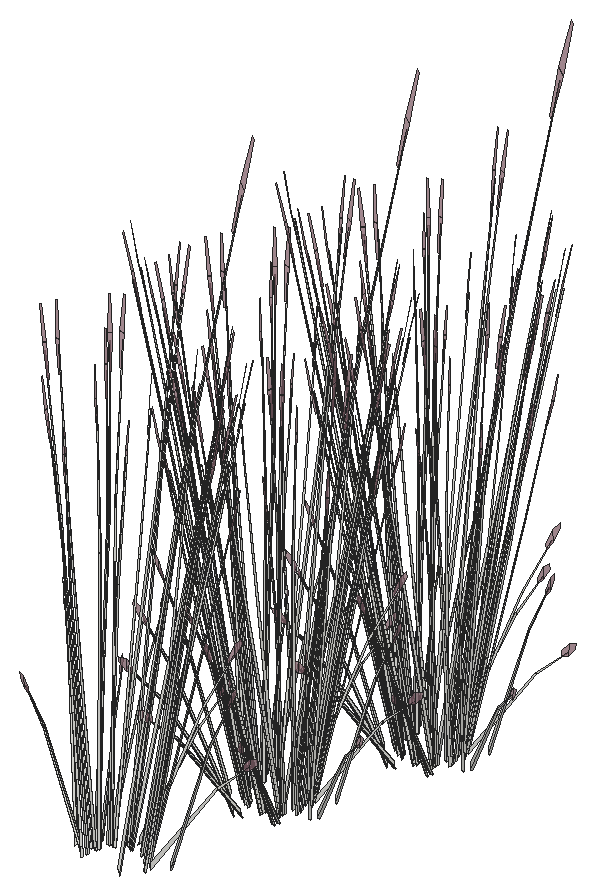
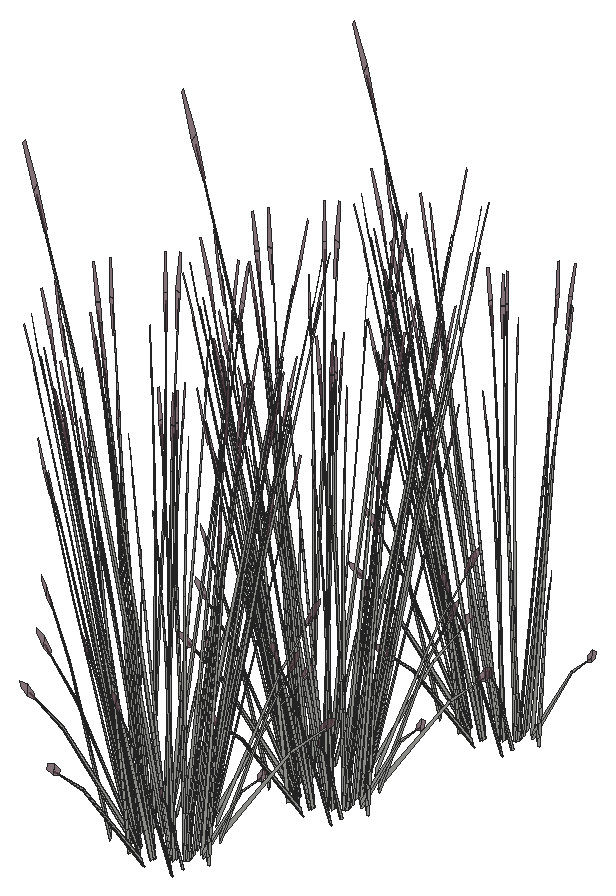
# SketchUp Ruby script. Lengths in inches.
U = 1.inch
M = Sketchup.active_model
def pt(a) = Geom::Point3d.new(a.map { |v| v * U })
def face(e, loops, mat)
  f = e.add_face(loops[0].map { |a| pt(a) })
  loops[1..].each { |l| e.add_face(l.map { |a| pt(a) }).erase! }
  f.material = f.back_material = mat if mat
  f
end
# faces: each face lists its corners as indices into pts; further lists are holes
def faces(e, pts, list, mat = nil) = list.each { |f| face(e, (f[0].is_a?(Array) ? f : [f]).map { |l| l.map { |i| pts[i] } }, mat) }
# xy, xz, yz: faces in a plane at the given z, y or x. An outline is a flat list of corners, or four numbers for a rectangle; further outlines are holes
def ring(l) = l.size == 4 ? [[l[0], l[1]], [l[2], l[1]], [l[2], l[3]], [l[0], l[3]]] : l.each_slice(2).to_a
def flat(e, list, mat, &to3) = list.each { |f| face(e, (f[0].is_a?(Array) ? f : [f]).map { |l| ring(l).map { |u, v| to3.(u, v) } }, mat) }
def xy(e, z, list, mat = nil) = flat(e, list, mat) { |x, y| [x, y, z] }
def xz(e, y, list, mat = nil) = flat(e, list, mat) { |x, z| [x, y, z] }
def yz(e, x, list, mat = nil) = flat(e, list, mat) { |y, z| [x, y, z] }
def lines(e, pts, list) = list.each { |a, b| e.add_line(pt(pts[a]), pt(pts[b])) }
# prism: a flat outline (further loops are holes) pulled along v
def prism(e, loops, v, mat = nil)
  f = face(e, loops, mat); d = Geom::Vector3d.new(v.map { |x| x * U })
  f.pushpull(f.normal.samedirection?(d) ? d.length : -d.length)
end
def box(e, o, s, mat = nil) = prism(e, [[o, [o[0] + s[0], o[1], o[2]], [o[0] + s[0], o[1] + s[1], o[2]], [o[0], o[1] + s[1], o[2]]]], [0, 0, s[2]], mat)
def at(x, y, z, deg = 0) = Geom::Transformation.translation(pt([x, y, z])) * Geom::Transformation.rotation(ORIGIN, Z_AXIS, deg.degrees)
def axes(o, x, y, z) = Geom::Transformation.new([*x, 0, *y, 0, *z, 0, *pt(o).to_a, 1])
def part(name) = M.definitions.add(name)
# library, detail: a bought-in or finely detailed component or shape, given as its bounding box
def library(name, o, s) = part(name).tap { |d| box(d.entities, o, s) }
def detail(e, o, s) = box(e.add_group.entities, o, s)
def put(e, d, t, mat = nil) = e.add_instance(d, t).tap { |i| i.material = mat if mat }
def group(e, t, mat = nil) = e.add_group.tap { |g| g.transformation = t; g.material = mat if mat }.entities
root = M.entities
M.materials.add("LightPink_Translucent").color = [144, 107, 117]
M.materials["LightPink_Translucent"].alpha = 0.75
c1 = part("blade")
p = [[2.15,0.21,22],[0,0.17,0],[0.09,0.45,0],[2.18,0.31,22],[2.29,0.31,22],[0.38,0.45,0],
  [2.48,0.24,33],[2.49,0.24,33],[2.48,0.22,33]]
faces(c1.entities,p,[[0,1,2,3],[4,5,2,3],[6,3,4,7],[8,0,3,6]])
c2 = part("seeds")
p = [[0.3,-0.1,1.38],[-0.01,-0.03,1.59],[-0.01,-0.03,0.03],[0.14,-0.07,-0.07],[0.29,-0.03,3],[0.15,0.01,3.11]]
faces(c2.entities,p,[[0,1,2,3],[1,0,4,5]],"LightPink_Translucent")
c3 = part("blade with seeds")
put(c3.entities,c1,at(0,0,0))
put(c3.entities,c2,axes([2.4,0.25,30.99],[1.5799,-0.05474,1.17369],[-0.12525,1.92788,0.29478],[-0.07173,-0.02425,1.56792]))
put(root,c3,axes([315.38,325.84,526.73],[-0.14195,0.49104,0.48003],[-0.46669,-0.16791,0.3958],[0.18353,-0.02951,0.9933]))
put(root,c3,axes([311.01,325.04,527.05],[0.41757,0.15024,0.35414],[-0.12179,0.4383,-0.4572],[-0.16812,0.04019,0.87481]))
put(root,c3,axes([316.22,327.43,526.71],[-0.04543,-0.04715,1.77383],[0.09938,-0.50538,-0.16761],[0.17896,-0.03229,0.31391]))
put(root,c3,axes([310.3,325.375,526.72],[-0.08205,0.06992,1.74944],[0.00698,0.51086,-0.27667],[-0.18807,0.06644,0.14031]))
put(root,c3,axes([310.83,324.89,527.03],[0.25281,0.48765,-0.1216],[-0.44869,0.23964,-0.67495],[-0.18908,0.06434,1.02557]))
put(root,c3,axes([314.64,326.99,527.03],[0.0269,-0.54769,-0.1216],[0.50939,0.01497,-0.67495],[0.19618,0.03804,1.02557]))
put(root,c3,axes([314.57,326.78,527.05],[-0.28589,-0.33718,0.35414],[0.32644,-0.31919,-0.4572],[0.16586,0.04856,0.87481]))
put(root,c3,axes([315.09,326.66,526.72],[0.10779,-0.00911,1.74944],[0.29564,-0.41839,-0.27667],[0.19172,0.05523,0.14031]))
put(root,c3,axes([310.78,326.25,526.73],[-0.12461,-0.49565,0.48003],[0.48882,-0.08602,0.3958],[-0.14406,0.11657,0.9933]))
put(root,c3,axes([310.68,326.16,526.73],[-0.34493,-0.22649,0.0643],[0.20082,-0.32253,0.50621],[-0.11059,0.10427,0.77189]))
put(root,c3,axes([311.08,326.09,527.05],[0.43736,-0.07697,0.35414],[0.11549,0.43998,-0.4572],[-0.12533,0.11818,0.87481]))
put(root,c3,axes([309.39,325.89,526.71],[0.06412,0.01444,1.77383],[0.19837,0.47583,-0.16761],[-0.13126,0.12489,0.31391]))
put(root,c3,axes([314.82,327.08,526.73],[-0.0253,0.40952,0.0643],[-0.38204,-0.01123,0.50621],[0.14634,0.04285,0.77189]))
put(root,c3,axes([314.86,326.95,526.73],[-0.37048,0.35486,0.48003],[-0.31952,-0.37685,0.3958],[0.17382,0.06546,0.9933]))
put(root,c3,axes([310.08,327.34,527.65],[0.44338,0.14375,-0.06488],[-0.13639,0.44245,-0.29416],[-0.07252,0.06718,0.97024]))
put(root,c3,axes([313.68,327.36,527.05],[-0.0776,-0.43378,0.35414],[0.44361,-0.11454,-0.4572],[0.11915,0.12431,0.87481]))
put(root,c3,axes([313.98,324.87,526.47],[-0.43417,-0.27982,1.38283],[0.45844,-0.43566,0.59665],[0.14008,0.26255,1.33663]))
put(root,c3,axes([310.85,326.05,527.03],[0.46478,0.29695,-0.1216],[-0.26776,0.43004,-0.67495],[-0.13131,0.14949,1.02557]))
put(root,c3,axes([313.64,327.59,527.03],[0.2994,-0.46097,-0.1216],[0.43359,0.26557,-0.67495],[0.15072,0.13024,1.02557]))
put(root,c3,axes([311.67,326.96,527.05],[0.33997,-0.28354,0.35414],[0.32182,0.32376,-0.4572],[-0.04897,0.1645,0.87481]))
put(root,c3,axes([313.25,327.97,526.71],[0.00149,-0.0652,1.77383],[0.43058,-0.28766,-0.16761],[0.14956,0.10267,0.31391]))
put(root,c3,axes([311.36,327.22,526.73],[-0.4129,-0.02509,0.0643],[0.01132,-0.37891,0.50621],[-0.04321,0.14514,0.77189]))
put(root,c3,axes([311.49,327.26,526.73],[-0.35779,-0.36745,0.48003],[0.37996,-0.3169,0.3958],[-0.066,0.17239,0.9933]))
put(root,c3,axes([312.62,327.43,527.05],[0.15148,-0.41415,0.35414],[0.44193,0.12079,-0.4572],[0.04052,0.16674,0.87481]))
put(root,c3,axes([313.75,327.75,526.73],[-0.22836,0.34211,0.0643],[-0.3252,-0.19918,0.50621],[0.10513,0.10968,0.77189]))
put(root,c3,axes([313.22,328.91,527.65],[0.34721,-0.30895,-0.06488],[0.31814,0.33837,-0.29416],[0.0224,0.09588,0.97024]))
put(root,c3,axes([313.85,327.66,526.73],[-0.49974,0.12359,0.48003],[-0.08673,-0.48481,0.3958],[0.11753,0.14288,0.9933]))
put(root,c3,axes([312.48,327.81,526.73],[-0.37023,0.18303,0.0643],[-0.18122,-0.33376,0.50621],[0.03575,0.14712,0.77189]))
put(root,c3,axes([310.32,327.28,526.72],[-0.01249,0.10657,1.74944],[0.35444,0.37075,-0.27667],[-0.09279,0.17532,0.14031]))
put(root,c3,axes([311.45,327.04,527.4],[0.55221,0.02668,-0.13498],[-0.01509,0.50521,-0.74919],[-0.03836,0.19458,1.13838]))
put(root,c3,axes([312.47,327.6,527.03],[0.49168,-0.25073,-0.1216],[0.24162,0.44501,-0.67495],[0.06487,0.18753,1.02557]))
put(root,c3,axes([312.61,327.77,527.0625],[-0.4951,-0.14079,0.53283],[0.1693,-0.46287,0.43934],[0.02975,0.18203,1.10256]))
put(root,c3,axes([310.28,328.375,526.71],[0.057,-0.03251,1.77383],[0.47114,0.21627,-0.16761],[-0.01107,0.18007,0.31391]))
put(root,c3,axes([315.61,335.45,526.72],[-0.07685,-0.07551,1.74944],[-0.51287,0.04787,-0.27667],[-0.08185,-0.1806,0.14031]))
put(root,c3,axes([312.36,328.6,526.72],[0.06369,0.08672,1.74944],[0.51399,0.03407,-0.27667],[0.05169,0.19126,0.14031]))
put(root,c3,axes([317.92,336.375,526.72],[-0.00485,-0.10718,1.74944],[-0.40965,-0.30977,-0.27667],[0.06333,-0.18778,0.14031]))
put(root,c3,axes([317.81,335.99,526.71],[-0.05103,0.04113,1.77383],[-0.49994,-0.13878,-0.16761],[-0.0181,-0.17951,0.31391]))
put(root,c3,axes([315.09,335.2,526.71],[-0.00937,0.06455,1.77383],[-0.46231,0.23427,-0.16761],[-0.13604,-0.11975,0.31391]))
put(root,c3,axes([314.98,336.35,527.09],[0.55971,-0.13842,0.53763],[0.09714,0.54299,0.4433],[-0.13164,-0.16003,1.11249]))
put(root,c3,axes([316.25,336.45,526.73],[0.4951,0.14079,0.48003],[-0.1693,0.46287,0.3958],[-0.02975,-0.18203,0.9933]))
put(root,c3,axes([316.39,336.61,527.03],[-0.49168,0.25073,-0.1216],[-0.24162,-0.44501,-0.67495],[-0.06487,-0.18753,1.02557]))
put(root,c3,axes([317.41,337.18,527.03],[-0.55221,-0.02668,-0.1216],[0.01509,-0.50521,-0.67495],[0.03836,-0.19458,1.02557]))
put(root,c3,axes([316.38,336.41,526.73],[0.37023,-0.18303,0.0643],[0.18122,0.33376,0.50621],[-0.03575,-0.14712,0.77189]))
put(root,c3,axes([315.11,336.46,526.73],[0.22836,-0.34211,0.0643],[0.3252,0.19918,0.50621],[-0.10513,-0.10968,0.77189]))
put(root,c3,axes([316.24,336.79,527.05],[-0.15148,0.41415,0.35414],[-0.44193,-0.12079,-0.4572],[-0.04052,-0.16674,0.87481]))
put(root,c3,axes([317.375,336.96,526.73],[0.35779,0.36745,0.48003],[-0.37996,0.3169,0.3958],[0.066,-0.17239,0.9933]))
put(root,c3,axes([315.22,336.43,527.43],[-0.33533,0.51628,-0.13619],[-0.48563,-0.29744,-0.75594],[-0.16881,-0.14586,1.14864]))
put(root,c3,axes([317.51,337,526.73],[0.4129,0.02509,0.0643],[-0.01132,0.37891,0.50621],[0.04321,-0.14514,0.77189]))
put(root,c3,axes([317.2,337.26,527.05],[-0.33997,0.28354,0.35414],[-0.32182,-0.32376,-0.4572],[0.04897,-0.1645,0.87481]))
put(root,c3,axes([313.93,336.28,526.72],[-0.10811,-0.0038,1.74944],[-0.34418,0.38014,-0.27667],[-0.18364,-0.07767,0.14031]))
put(root,c3,axes([318.01,338.17,527.03],[-0.46478,-0.29695,-0.1216],[0.26776,-0.43004,-0.67495],[0.13131,-0.14949,1.02557]))
put(root,c3,axes([315.18,336.86,527.05],[0.0776,0.43378,0.35414],[-0.44361,0.11454,-0.4572],[-0.11915,-0.12431,0.87481]))
put(root,c3,axes([313.85,337.14,527.09],[0.41494,-0.39744,0.53763],[0.35786,0.42207,0.4433],[-0.19468,-0.07331,1.11249]))
put(root,c3,axes([319.16,338.04,526.71],[-0.06563,-0.00409,1.77383],[-0.27252,-0.43825,-0.16761],[0.10944,-0.1441,0.31391]))
put(root,c3,axes([314.04,337.14,526.73],[0.0253,-0.40952,0.0643],[0.38204,0.01123,0.50621],[-0.14634,-0.04285,0.77189]))
put(root,c3,axes([317.79,338.13,527.05],[-0.43736,0.07697,0.35414],[-0.11549,-0.43998,-0.4572],[0.12533,-0.11818,0.87481]))
put(root,c3,axes([318.18,338.0625,526.73],[0.34493,0.22649,0.0643],[-0.20082,0.32253,0.50621],[0.11059,-0.10427,0.77189]))
put(root,c3,axes([318.09,337.97,526.73],[0.12461,0.49565,0.48003],[-0.48882,0.08602,0.3958],[0.14406,-0.11657,0.9933]))
put(root,c3,axes([319.41,338.57,526.72],[0.06972,-0.08203,1.74944],[-0.08924,-0.50318,-0.27667],[0.17494,-0.0954,0.14031]))
put(root,c3,axes([313.51,336.6,526.71],[0.03725,0.05374,1.77383],[-0.17957,0.48312,-0.16761],[-0.18186,0.0035,0.31391]))
put(root,c3,axes([314.3,337.44,527.05],[0.28589,0.33718,0.35414],[-0.32644,0.31919,-0.4572],[-0.16586,-0.04856,0.87481]))
put(root,c3,axes([314.22,337.23,527.03],[-0.0269,0.54769,-0.1216],[-0.50939,-0.01497,-0.67495],[-0.19618,-0.03804,1.02557]))
put(root,c3,axes([318.03,339.33,527.03],[-0.25281,-0.48765,-0.1216],[0.44869,-0.23964,-0.67495],[0.18908,-0.06434,1.02557]))
put(root,c3,axes([317.86,339.18,527.05],[-0.41757,-0.15024,0.35414],[0.12179,-0.4383,-0.4572],[0.16812,-0.04019,0.87481]))
put(root,c3,axes([313.49,338.38,526.73],[0.14195,-0.49104,0.48003],[0.46669,0.16791,0.3958],[-0.18353,0.02951,0.9933]))
put(root,c3,axes([313.45,338.25,526.73],[-0.18454,-0.3672,0.0643],[0.33652,-0.17973,0.50621],[-0.14834,0.03546,0.77189]))
put(root,c3,axes([318.24,339.32,526.73],[0.18454,0.3672,0.0643],[-0.33652,0.17973,0.50621],[0.14834,-0.03546,0.77189]))
put(root,c3,axes([318.2,339.19,526.73],[-0.14195,0.49104,0.48003],[-0.46669,-0.16791,0.3958],[0.18353,-0.02951,0.9933]))
put(root,c3,axes([313.83,338.39,527.05],[0.41757,0.15024,0.35414],[-0.12179,0.4383,-0.4572],[-0.16812,0.04019,0.87481]))
put(root,c3,axes([319.04,340.78,526.71],[-0.04543,-0.04715,1.77383],[0.09938,-0.50538,-0.16761],[0.17896,-0.03229,0.31391]))
put(root,c3,axes([313.125,338.73,526.72],[-0.08205,0.06992,1.74944],[0.00698,0.51086,-0.27667],[-0.18807,0.06644,0.14031]))
put(root,c3,axes([313.65,338.24,527.03],[0.25281,0.48765,-0.1216],[-0.44869,0.23964,-0.67495],[-0.18908,0.06434,1.02557]))
put(root,c3,axes([317.47,340.34,527.03],[0.0269,-0.54769,-0.1216],[0.50939,0.01497,-0.67495],[0.19618,0.03804,1.02557]))
put(root,c3,axes([317.39,340.13,527.05],[-0.28589,-0.33718,0.35414],[0.32644,-0.31919,-0.4572],[0.16586,0.04856,0.87481]))
put(root,c3,axes([317.91,340.02,526.72],[0.10779,-0.00911,1.74944],[0.29564,-0.41839,-0.27667],[0.19172,0.05523,0.14031]))
put(root,c3,axes([313.6,339.61,526.73],[-0.12461,-0.49565,0.48003],[0.48882,-0.08602,0.3958],[-0.14406,0.11657,0.9933]))
put(root,c3,axes([313.5,339.51,526.73],[-0.34493,-0.22649,0.0643],[0.20082,-0.32253,0.50621],[-0.11059,0.10427,0.77189]))
put(root,c3,axes([313.9,339.44,527.05],[0.43736,-0.07697,0.35414],[0.11549,0.43998,-0.4572],[-0.12533,0.11818,0.87481]))
put(root,c3,axes([312.21,339.25,526.71],[0.06412,0.01444,1.77383],[0.19837,0.47583,-0.16761],[-0.13126,0.12489,0.31391]))
put(root,c3,axes([317.65,340.44,526.73],[-0.0253,0.40952,0.0643],[-0.38204,-0.01123,0.50621],[0.14634,0.04285,0.77189]))
put(root,c3,axes([317.68,340.3,526.73],[-0.37048,0.35486,0.48003],[-0.31952,-0.37685,0.3958],[0.17382,0.06546,0.9933]))
put(root,c3,axes([312.91,340.69,527.65],[0.44338,0.14375,-0.06488],[-0.13639,0.44245,-0.29416],[-0.07252,0.06718,0.97024]))
put(root,c3,axes([316.5,340.72,527.05],[-0.0776,-0.43378,0.35414],[0.44361,-0.11454,-0.4572],[0.11915,0.12431,0.87481]))
put(root,c3,axes([316.8,338.22,526.47],[-0.43417,-0.27982,1.38283],[0.45844,-0.43566,0.59665],[0.14008,0.26255,1.33663]))
put(root,c3,axes([313.67,339.4,527.03],[0.46478,0.29695,-0.1216],[-0.26776,0.43004,-0.67495],[-0.13131,0.14949,1.02557]))
put(root,c3,axes([316.46,340.94,527.03],[0.2994,-0.46097,-0.1216],[0.43359,0.26557,-0.67495],[0.15072,0.13024,1.02557]))
put(root,c3,axes([314.49,340.32,527.05],[0.33997,-0.28354,0.35414],[0.32182,0.32376,-0.4572],[-0.04897,0.1645,0.87481]))
put(root,c3,axes([316.07,341.32,526.71],[0.00149,-0.0652,1.77383],[0.43058,-0.28766,-0.16761],[0.14956,0.10267,0.31391]))
put(root,c3,axes([314.18,340.57,526.73],[-0.4129,-0.02509,0.0643],[0.01132,-0.37891,0.50621],[-0.04321,0.14514,0.77189]))
put(root,c3,axes([314.3125,340.61,526.73],[-0.35779,-0.36745,0.48003],[0.37996,-0.3169,0.3958],[-0.066,0.17239,0.9933]))
put(root,c3,axes([319.28,346.52,526.72],[-0.07685,-0.07551,1.74944],[-0.51287,0.04787,-0.27667],[-0.08185,-0.1806,0.14031]))
put(root,c3,axes([315.44,340.78,527.05],[0.15148,-0.41415,0.35414],[0.44193,0.12079,-0.4572],[0.04052,0.16674,0.87481]))
put(root,c3,axes([316.57,341.11,526.73],[-0.22836,0.34211,0.0643],[-0.3252,-0.19918,0.50621],[0.10513,0.10968,0.77189]))
put(root,c3,axes([316.04,342.26,527.65],[0.34721,-0.30895,-0.06488],[0.31814,0.33837,-0.29416],[0.0224,0.09588,0.97024]))
put(root,c3,axes([316.67,341.01,526.73],[-0.49974,0.12359,0.48003],[-0.08673,-0.48481,0.3958],[0.11753,0.14288,0.9933]))
put(root,c3,axes([321.59,347.44,526.72],[-0.00485,-0.10718,1.74944],[-0.40965,-0.30977,-0.27667],[0.06333,-0.18778,0.14031]))
put(root,c3,axes([321.48,347.06,526.71],[-0.05103,0.04113,1.77383],[-0.49994,-0.13878,-0.16761],[-0.0181,-0.17951,0.31391]))
put(root,c3,axes([315.31,341.16,526.73],[-0.37023,0.18303,0.0643],[-0.18122,-0.33376,0.50621],[0.03575,0.14712,0.77189]))
put(root,c3,axes([313.14,340.64,526.72],[-0.01249,0.10657,1.74944],[0.35444,0.37075,-0.27667],[-0.09279,0.17532,0.14031]))
put(root,c3,axes([314.27,340.4,527.4],[0.55221,0.02668,-0.13498],[-0.01509,0.50521,-0.74919],[-0.03836,0.19458,1.13838]))
put(root,c3,axes([315.29,340.96,527.03],[0.49168,-0.25073,-0.1216],[0.24162,0.44501,-0.67495],[0.06487,0.18753,1.02557]))
put(root,c3,axes([315.4375,341.125,527.0625],[-0.4951,-0.14079,0.53283],[0.1693,-0.46287,0.43934],[0.02975,0.18203,1.10256]))
put(root,c3,axes([318.76,346.27,526.71],[-0.00937,0.06455,1.77383],[-0.46231,0.23427,-0.16761],[-0.13604,-0.11975,0.31391]))
put(root,c3,axes([318.66,347.41,527.09],[0.55971,-0.13842,0.53763],[0.09714,0.54299,0.4433],[-0.13164,-0.16003,1.11249]))
put(root,c3,axes([319.92,347.51,526.73],[0.4951,0.14079,0.48003],[-0.1693,0.46287,0.3958],[-0.02975,-0.18203,0.9933]))
put(root,c3,axes([320.0625,347.68,527.03],[-0.49168,0.25073,-0.1216],[-0.24162,-0.44501,-0.67495],[-0.06487,-0.18753,1.02557]))
put(root,c3,axes([321.09,348.24,527.03],[-0.55221,-0.02668,-0.1216],[0.01509,-0.50521,-0.67495],[0.03836,-0.19458,1.02557]))
put(root,c3,axes([320.05,347.48,526.73],[0.37023,-0.18303,0.0643],[0.18122,0.33376,0.50621],[-0.03575,-0.14712,0.77189]))
put(root,c3,axes([313.1,341.73,526.71],[0.057,-0.03251,1.77383],[0.47114,0.21627,-0.16761],[-0.01107,0.18007,0.31391]))
put(root,c3,axes([318.78,347.53,526.73],[0.22836,-0.34211,0.0643],[0.3252,0.19918,0.50621],[-0.10513,-0.10968,0.77189]))
put(root,c3,axes([319.92,347.85,527.05],[-0.15148,0.41415,0.35414],[-0.44193,-0.12079,-0.4572],[-0.04052,-0.16674,0.87481]))
put(root,c3,axes([321.05,348.03,526.73],[0.35779,0.36745,0.48003],[-0.37996,0.3169,0.3958],[0.066,-0.17239,0.9933]))
put(root,c3,axes([318.89,347.49,527.43],[-0.33533,0.51628,-0.13619],[-0.48563,-0.29744,-0.75594],[-0.16881,-0.14586,1.14864]))
put(root,c3,axes([315.18,341.95,526.72],[0.06369,0.08672,1.74944],[0.51399,0.03407,-0.27667],[0.05169,0.19126,0.14031]))
put(root,c3,axes([321.18,348.0625,526.73],[0.4129,0.02509,0.0643],[-0.01132,0.37891,0.50621],[0.04321,-0.14514,0.77189]))
put(root,c3,axes([320.87,348.32,527.05],[-0.33997,0.28354,0.35414],[-0.32182,-0.32376,-0.4572],[0.04897,-0.1645,0.87481]))
put(root,c3,axes([317.6,347.35,526.72],[-0.10811,-0.0038,1.74944],[-0.34418,0.38014,-0.27667],[-0.18364,-0.07767,0.14031]))
put(root,c3,axes([321.6875,349.24,527.03],[-0.46478,-0.29695,-0.1216],[0.26776,-0.43004,-0.67495],[0.13131,-0.14949,1.02557]))
put(root,c3,axes([318.86,347.92,527.05],[0.0776,0.43378,0.35414],[-0.44361,0.11454,-0.4572],[-0.11915,-0.12431,0.87481]))
put(root,c3,axes([317.52,348.21,527.09],[0.41494,-0.39744,0.53763],[0.35786,0.42207,0.4433],[-0.19468,-0.07331,1.11249]))
put(root,c3,axes([322.83,349.11,526.71],[-0.06563,-0.00409,1.77383],[-0.27252,-0.43825,-0.16761],[0.10944,-0.1441,0.31391]))
put(root,c3,axes([317.71,348.2,526.73],[0.0253,-0.40952,0.0643],[0.38204,0.01123,0.50621],[-0.14634,-0.04285,0.77189]))
put(root,c3,axes([321.46,349.2,527.05],[-0.43736,0.07697,0.35414],[-0.11549,-0.43998,-0.4572],[0.12533,-0.11818,0.87481]))
put(root,c3,axes([321.86,349.13,526.73],[0.34493,0.22649,0.0643],[-0.20082,0.32253,0.50621],[0.11059,-0.10427,0.77189]))
put(root,c3,axes([321.76,349.03,526.73],[0.12461,0.49565,0.48003],[-0.48882,0.08602,0.3958],[0.14406,-0.11657,0.9933]))
put(root,c3,axes([323.08,349.63,526.72],[0.06972,-0.08203,1.74944],[-0.08924,-0.50318,-0.27667],[0.17494,-0.0954,0.14031]))
put(root,c3,axes([317.1875,347.67,526.71],[0.03725,0.05374,1.77383],[-0.17957,0.48312,-0.16761],[-0.18186,0.0035,0.31391]))
put(root,c3,axes([317.97,348.51,527.05],[0.28589,0.33718,0.35414],[-0.32644,0.31919,-0.4572],[-0.16586,-0.04856,0.87481]))
put(root,c3,axes([317.89,348.29,527.03],[-0.0269,0.54769,-0.1216],[-0.50939,-0.01497,-0.67495],[-0.19618,-0.03804,1.02557]))
put(root,c3,axes([321.71,350.4,527.03],[-0.25281,-0.48765,-0.1216],[0.44869,-0.23964,-0.67495],[0.18908,-0.06434,1.02557]))
put(root,c3,axes([321.53,350.25,527.05],[-0.41757,-0.15024,0.35414],[0.12179,-0.4383,-0.4572],[0.16812,-0.04019,0.87481]))
put(root,c3,axes([317.16,349.45,526.73],[0.14195,-0.49104,0.48003],[0.46669,0.16791,0.3958],[-0.18353,0.02951,0.9933]))
put(root,c3,axes([317.12,349.32,526.73],[-0.18454,-0.3672,0.0643],[0.33652,-0.17973,0.50621],[-0.14834,0.03546,0.77189]))
put(root,c3,axes([321.91,350.39,526.73],[0.18454,0.3672,0.0643],[-0.33652,0.17973,0.50621],[0.14834,-0.03546,0.77189]))
put(root,c3,axes([321.87,350.26,526.73],[-0.14195,0.49104,0.48003],[-0.46669,-0.16791,0.3958],[0.18353,-0.02951,0.9933]))
put(root,c3,axes([317.5,349.45,527.05],[0.41757,0.15024,0.35414],[-0.12179,0.4383,-0.4572],[-0.16812,0.04019,0.87481]))
put(root,c3,axes([322.71,351.85,526.71],[-0.04543,-0.04715,1.77383],[0.09938,-0.50538,-0.16761],[0.17896,-0.03229,0.31391]))
put(root,c3,axes([316.8,349.79,526.72],[-0.08205,0.06992,1.74944],[0.00698,0.51086,-0.27667],[-0.18807,0.06644,0.14031]))
put(root,c3,axes([317.33,349.31,527.03],[0.25281,0.48765,-0.1216],[-0.44869,0.23964,-0.67495],[-0.18908,0.06434,1.02557]))
put(root,c3,axes([321.14,351.41,527.03],[0.0269,-0.54769,-0.1216],[0.50939,0.01497,-0.67495],[0.19618,0.03804,1.02557]))
put(root,c3,axes([321.06,351.2,527.05],[-0.28589,-0.33718,0.35414],[0.32644,-0.31919,-0.4572],[0.16586,0.04856,0.87481]))
put(root,c3,axes([321.58,351.08,526.72],[0.10779,-0.00911,1.74944],[0.29564,-0.41839,-0.27667],[0.19172,0.05523,0.14031]))
put(root,c3,axes([317.27,350.67,526.73],[-0.12461,-0.49565,0.48003],[0.48882,-0.08602,0.3958],[-0.14406,0.11657,0.9933]))
put(root,c3,axes([317.17,350.58,526.73],[-0.34493,-0.22649,0.0643],[0.20082,-0.32253,0.50621],[-0.11059,0.10427,0.77189]))
put(root,c3,axes([317.57,350.51,527.05],[0.43736,-0.07697,0.35414],[0.11549,0.43998,-0.4572],[-0.12533,0.11818,0.87481]))
put(root,c3,axes([315.89,350.3125,526.71],[0.06412,0.01444,1.77383],[0.19837,0.47583,-0.16761],[-0.13126,0.12489,0.31391]))
put(root,c3,axes([321.32,351.5,526.73],[-0.0253,0.40952,0.0643],[-0.38204,-0.01123,0.50621],[0.14634,0.04285,0.77189]))
put(root,c3,axes([321.35,351.37,526.73],[-0.37048,0.35486,0.48003],[-0.31952,-0.37685,0.3958],[0.17382,0.06546,0.9933]))
put(root,c3,axes([316.58,351.76,527.65],[0.44338,0.14375,-0.06488],[-0.13639,0.44245,-0.29416],[-0.07252,0.06718,0.97024]))
put(root,c3,axes([320.18,351.78,527.05],[-0.0776,-0.43378,0.35414],[0.44361,-0.11454,-0.4572],[0.11915,0.12431,0.87481]))
put(root,c3,axes([320.47,349.29,526.47],[-0.43417,-0.27982,1.38283],[0.45844,-0.43566,0.59665],[0.14008,0.26255,1.33663]))
put(root,c3,axes([317.34,350.47,527.03],[0.46478,0.29695,-0.1216],[-0.26776,0.43004,-0.67495],[-0.13131,0.14949,1.02557]))
put(root,c3,axes([320.13,352.01,527.03],[0.2994,-0.46097,-0.1216],[0.43359,0.26557,-0.67495],[0.15072,0.13024,1.02557]))
put(root,c3,axes([318.16,351.38,527.05],[0.33997,-0.28354,0.35414],[0.32182,0.32376,-0.4572],[-0.04897,0.1645,0.87481]))
put(root,c3,axes([319.74,352.39,526.71],[0.00149,-0.0652,1.77383],[0.43058,-0.28766,-0.16761],[0.14956,0.10267,0.31391]))
put(root,c3,axes([317.85,351.64,526.73],[-0.4129,-0.02509,0.0643],[0.01132,-0.37891,0.50621],[-0.04321,0.14514,0.77189]))
put(root,c3,axes([317.98,351.68,526.73],[-0.35779,-0.36745,0.48003],[0.37996,-0.3169,0.3958],[-0.066,0.17239,0.9933]))
put(root,c3,axes([319.11,351.85,527.05],[0.15148,-0.41415,0.35414],[0.44193,0.12079,-0.4572],[0.04052,0.16674,0.87481]))
put(root,c3,axes([320.25,352.17,526.73],[-0.22836,0.34211,0.0643],[-0.3252,-0.19918,0.50621],[0.10513,0.10968,0.77189]))
put(root,c3,axes([319.71,353.33,527.65],[0.34721,-0.30895,-0.06488],[0.31814,0.33837,-0.29416],[0.0224,0.09588,0.97024]))
put(root,c3,axes([320.34,352.08,526.73],[-0.49974,0.12359,0.48003],[-0.08673,-0.48481,0.3958],[0.11753,0.14288,0.9933]))
put(root,c3,axes([318.98,352.23,526.73],[-0.37023,0.18303,0.0643],[-0.18122,-0.33376,0.50621],[0.03575,0.14712,0.77189]))
put(root,c3,axes([316.8125,351.7,526.72],[-0.01249,0.10657,1.74944],[0.35444,0.37075,-0.27667],[-0.09279,0.17532,0.14031]))
put(root,c3,axes([317.94,351.46,527.4],[0.55221,0.02668,-0.13498],[-0.01509,0.50521,-0.74919],[-0.03836,0.19458,1.13838]))
put(root,c3,axes([318.97,352.02,527.03],[0.49168,-0.25073,-0.1216],[0.24162,0.44501,-0.67495],[0.06487,0.18753,1.02557]))
put(root,c3,axes([319.11,352.19,527.0625],[-0.4951,-0.14079,0.53283],[0.1693,-0.46287,0.43934],[0.02975,0.18203,1.10256]))
put(root,c3,axes([316.77,352.79,526.71],[0.057,-0.03251,1.77383],[0.47114,0.21627,-0.16761],[-0.01107,0.18007,0.31391]))
put(root,c3,axes([318.85,353.02,526.72],[0.06369,0.08672,1.74944],[0.51399,0.03407,-0.27667],[0.05169,0.19126,0.14031]))
